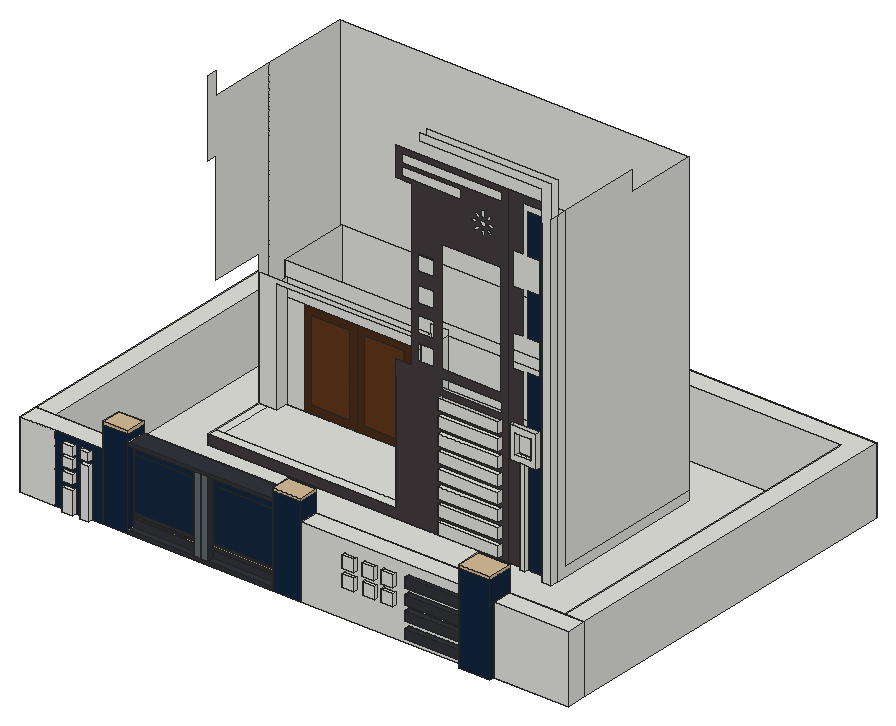
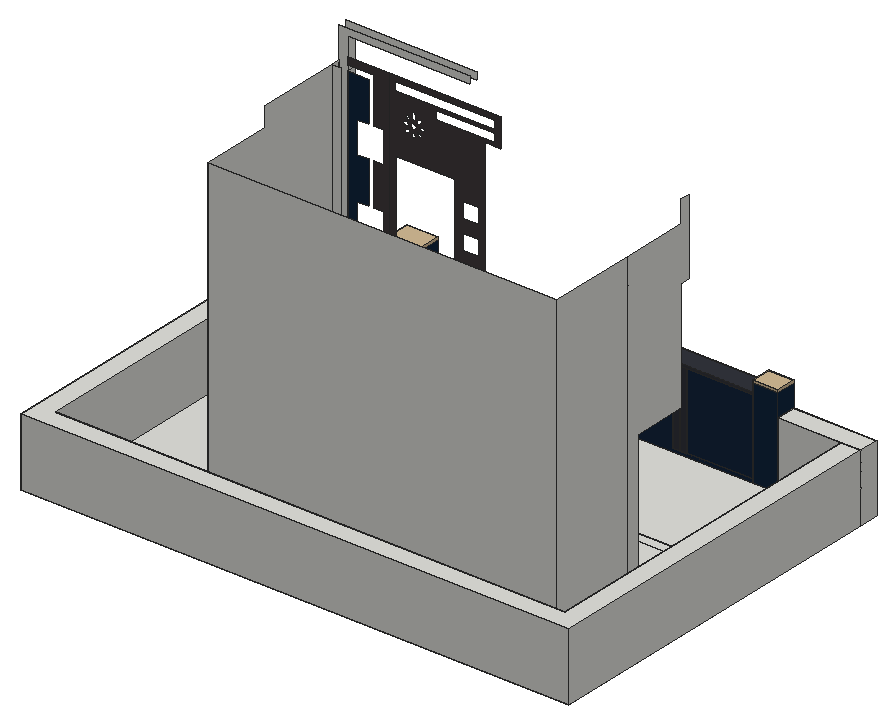
# SketchUp Ruby script. Lengths in inches.
U = 1.inch
M = Sketchup.active_model
def pt(a) = Geom::Point3d.new(a.map { |v| v * U })
def face(e, loops, mat)
  f = e.add_face(loops[0].map { |a| pt(a) })
  loops[1..].each { |l| e.add_face(l.map { |a| pt(a) }).erase! }
  f.material = f.back_material = mat if mat
  f
end
# faces: each face lists its corners as indices into pts; further lists are holes
def faces(e, pts, list, mat = nil) = list.each { |f| face(e, (f[0].is_a?(Array) ? f : [f]).map { |l| l.map { |i| pts[i] } }, mat) }
# xy, xz, yz: faces in a plane at the given z, y or x. An outline is a flat list of corners, or four numbers for a rectangle; further outlines are holes
def ring(l) = l.size == 4 ? [[l[0], l[1]], [l[2], l[1]], [l[2], l[3]], [l[0], l[3]]] : l.each_slice(2).to_a
def flat(e, list, mat, &to3) = list.each { |f| face(e, (f[0].is_a?(Array) ? f : [f]).map { |l| ring(l).map { |u, v| to3.(u, v) } }, mat) }
def xy(e, z, list, mat = nil) = flat(e, list, mat) { |x, y| [x, y, z] }
def xz(e, y, list, mat = nil) = flat(e, list, mat) { |x, z| [x, y, z] }
def yz(e, x, list, mat = nil) = flat(e, list, mat) { |y, z| [x, y, z] }
def lines(e, pts, list) = list.each { |a, b| e.add_line(pt(pts[a]), pt(pts[b])) }
# prism: a flat outline (further loops are holes) pulled along v
def prism(e, loops, v, mat = nil)
  f = face(e, loops, mat); d = Geom::Vector3d.new(v.map { |x| x * U })
  f.pushpull(f.normal.samedirection?(d) ? d.length : -d.length)
end
def box(e, o, s, mat = nil) = prism(e, [[o, [o[0] + s[0], o[1], o[2]], [o[0] + s[0], o[1] + s[1], o[2]], [o[0], o[1] + s[1], o[2]]]], [0, 0, s[2]], mat)
def at(x, y, z, deg = 0) = Geom::Transformation.translation(pt([x, y, z])) * Geom::Transformation.rotation(ORIGIN, Z_AXIS, deg.degrees)
def axes(o, x, y, z) = Geom::Transformation.new([*x, 0, *y, 0, *z, 0, *pt(o).to_a, 1])
def part(name) = M.definitions.add(name)
# library, detail: a bought-in or finely detailed component or shape, given as its bounding box
def library(name, o, s) = part(name).tap { |d| box(d.entities, o, s) }
def detail(e, o, s) = box(e.add_group.entities, o, s)
def put(e, d, t, mat = nil) = e.add_instance(d, t).tap { |i| i.material = mat if mat }
def group(e, t, mat = nil) = e.add_group.tap { |g| g.transformation = t; g.material = mat if mat }.entities
root = M.entities
M.materials.add("[Asphalt New]").color = [96, 86, 89]
M.materials.add("[Asphalt New]1").color = [67, 60, 62]
M.materials.add("[Carrera Marble]").color = [19, 39, 63]
M.materials.add("[Carrera Marble]1").color = [22, 39, 63]
M.materials.add("[Formica Beige]").color = [211, 187, 149]
M.materials.add("[Formica Laminate Dark]").color = [50, 53, 60]
M.materials.add("[Formica Speckled Grey]").color = [94, 105, 111]
M.materials.add("[Wood Cherry Original]").color = [96, 54, 26]
M.materials.add("[Wood Veneer 01]").color = [76, 44, 23]
xy(root,-39.0625,[[433.06,0,463.46,24.21],[44.56,0.625,54.43,5],[61.81,0.625,70.31,5],[0,5,81.17,24.21],[81.17,5,105.62,24.21],
  [105.62,5,247.01,24.21],[247.01,5,274.33,24.21],[274.33,5,433.06,24.21],[463.46,5,536.875,24.21],[0,24.21,0,381.625,536.875,381.625,536.875,24.21,517.66,24.21,517.66,362.41,19.21,362.41,19.21,24.21],
  [[19.21,24.21,517.66,362.41],[374.5,148.04,379.09,152.35]],[399.65,143.85,408.27,152.35],[374.5,148.04,379.09,152.35],[65.99,152.35,408.27,313.28]])
xy(root,-35.83,[[294.43,147.85,353.36,152.35]])
xy(root,-35.625,[[169.86,5,176.72,24.21],[176.72,5,183.58,24.21],[105.62,11.68,169.86,24.21]])
xy(root,-35.625,[[105.62,5,169.86,11.68],[183.58,5,247.01,11.68]],"[Formica Laminate Dark]")
xy(root,-32.16,[[380.62,0,433.06,5]],"[Formica Laminate Dark]")
xy(root,-30.0625,[[65.99,152.35,249.72,161.35],[399.27,161.35,399.27,304.28,74.99,304.28,74.99,226.93,65.99,226.93,65.99,313.28,408.27,313.28,408.27,161.35],[65.99,161.35,74.99,214.25],[74.99,161.35,399.27,161.35,399.27,226.93,241.35,226.93,241.35,214.25,224.39,214.25,224.39,226.93,83.43,226.93,83.43,214.25,74.99,214.25],[65.99,214.25,74.99,226.93],
  [74.99,214.25,83.43,226.93],[224.39,214.25,241.35,226.93],[74.99,226.93,399.27,234.75],[74.99,234.75,399.27,304.28]])
xy(root,-25.15,[[294.43,147.85,353.36,152.35]])
xy(root,-23.16,[[380.62,0,433.06,5]],"[Formica Laminate Dark]")
xy(root,-20.02,[[294.43,147.85,353.36,152.35]])
xy(root,-17.375,[[44.56,0.625,54.43,5]])
xy(root,-16.35,[[380.62,0,433.06,5]],"[Formica Laminate Dark]")
xy(root,-12.27,[[44.06,0.625,54.43,5]])
xy(root,-9.47,[[317.33,1.5625,329.02,5],[337.77,1.5625,349.45,5],[355.89,1.5625,367.58,5]])
xy(root,-9.33,[[294.43,147.85,353.36,152.35]])
xy(root,-7.35,[[380.62,0,433.06,5]],"[Formica Laminate Dark]")
xy(root,-4.33,[[294.43,147.85,353.36,152.35]])
xy(root,-3.45,[[44.06,0.625,54.43,5]])
xy(root,-2.54,[[380.62,0,433.06,5]],"[Formica Laminate Dark]")
xy(root,1.11,[[44.06,0.625,54.43,5]])
xy(root,2.22,[[317.33,1.5625,329.02,5],[337.77,1.5625,349.45,5],[355.89,1.5625,367.58,5]])
xy(root,6.35,[[294.43,147.85,353.36,152.35]])
xy(root,6.46,[[380.62,0,433.06,5]],"[Formica Laminate Dark]")
xy(root,7.16,[[317.33,1.5625,329.02,5],[337.45,1.5625,349.14,5],[355.95,1.5625,367.64,5]])
xy(root,9.75,[[61.81,0.625,70.31,5]])
xy(root,9.92,[[44.06,0.625,54.43,5]])
xy(root,11.17,[[294.43,147.85,353.36,152.35]])
xy(root,12.67,[[44.06,0.625,54.43,5]])
xy(root,12.9,[[380.62,0,433.06,5]],"[Formica Laminate Dark]")
xy(root,13.2,[[61.37,0.625,69.68,5]])
xy(root,18.84,[[317.33,1.5625,329.02,5],[337.45,1.5625,349.14,5],[355.95,1.5625,367.64,5]])
xy(root,21.48,[[44.06,0.625,54.43,5]])
xy(root,21.51,[[61.37,0.625,69.68,5]])
xy(root,21.85,[[294.43,147.85,353.36,152.35]])
xy(root,21.9,[[380.62,0,433.06,5]],"[Formica Laminate Dark]")
xy(root,26.67,[[294.43,147.85,353.36,152.35]])
xy(root,27,[[0,5,81.17,24.21],[463.46,5,536.875,24.21],[0,24.21,19.21,24.21,19.21,362.41,517.66,362.41,517.66,24.21,536.875,24.21,536.875,381.625,0,381.625]])
xy(root,30.5625,[[274.33,5,433.06,24.21]])
xy(root,37.35,[[294.43,147.85,353.36,152.35]])
xy(root,38.57,[[105.62,5,169.86,11.68],[176.72,5,183.58,24.21],[183.58,5,247.01,11.68]])
xy(root,41.45,[[105.62,5,247.01,24.21]],"[Formica Laminate Dark]")
xy(root,42.17,[[294.43,147.85,353.36,152.35]])
xy(root,48.5625,[[433.06,0,463.46,24.21],[81.17,5,105.62,24.21],[247.01,5,274.33,24.21]])
xy(root,51.5,[[433.06,0,463.46,24.21],[81.17,5,105.62,24.21],[247.01,5,274.33,24.21]],"[Formica Beige]")
xy(root,52.85,[[294.43,147.85,353.36,152.35]])
xy(root,54.85,[[364.57,148.04,374.5,152.35],[374.5,148.04,379.09,152.35],[379.09,148.04,390.63,152.35]])
xy(root,57.67,[[294.43,147.85,353.36,152.35]])
xy(root,60.36,[[370.09,148.04,374.5,152.35],[374.5,148.04,379.09,152.35],[379.09,148.04,385.11,152.35]])
xy(root,68.35,[[294.43,147.85,353.36,152.35]])
xy(root,73.17,[[294.43,147.85,353.36,152.35]])
xz(root,0,[[433.06,-39.0625,463.46,48.5625]],"[Carrera Marble]")
xz(root,0,[[433.06,48.5625,463.46,51.5]],"[Formica Beige]")
xz(root,0,[[380.62,-32.16,433.06,-23.16],[380.62,-16.35,433.06,-7.35],[380.62,-2.54,433.06,6.46],[380.62,12.9,433.06,21.9]],"[Formica Laminate Dark]")
xz(root,0.625,[[44.56,-39.0625,54.43,-17.375],[61.81,-39.0625,70.31,9.75],[44.06,-12.27,54.43,-3.45],[44.06,1.11,54.43,9.92],[44.06,12.67,54.43,21.48],
  [61.37,13.2,69.68,21.51]])
xz(root,1.5625,[[317.33,-9.47,329.02,2.22],[337.77,-9.47,349.45,2.22],[355.89,-9.47,367.58,2.22],[317.33,7.16,329.02,18.84],[337.45,7.16,349.14,18.84],
  [355.95,7.16,367.64,18.84]])
xz(root,5,[[0,-39.0625,33.95,27],[44.56,-39.0625,54.43,-17.375],[61.81,-39.0625,70.31,9.75],[[274.33,-39.0625,433.06,-39.0625,433.06,-32.16,380.62,-32.16,380.62,-23.16,433.06,-23.16,433.06,-16.35,380.62,-16.35,380.62,-7.35,433.06,-7.35,433.06,-2.54,380.62,-2.54,380.62,6.46,433.06,6.46,433.06,12.9,380.62,12.9,380.62,21.9,433.06,21.9,433.06,30.5625,274.33,30.5625],[317.33,7.16,329.02,18.84],[337.45,7.16,349.14,18.84],[355.95,7.16,367.64,18.84],[317.33,-9.47,329.02,2.22],[337.77,-9.47,349.45,2.22],[355.89,-9.47,367.58,2.22]],[463.46,-39.0625,536.875,27],
  [44.06,-12.27,54.43,-3.45],[317.33,-9.47,329.02,2.22],[337.77,-9.47,349.45,2.22],[355.89,-9.47,367.58,2.22],[44.06,1.11,54.43,9.92],
  [317.33,7.16,329.02,18.84],[337.45,7.16,349.14,18.84],[355.95,7.16,367.64,18.84],[44.06,12.67,54.43,21.48],[61.37,13.2,69.68,21.51]])
xz(root,5,[[[33.95,-39.0625,44.56,-39.0625,44.56,-17.375,54.43,-17.375,54.43,-39.0625,61.81,-39.0625,61.81,9.75,70.31,9.75,70.31,-39.0625,81.17,-39.0625,81.17,27,33.95,27],[44.06,-12.27,54.43,-3.45],[44.06,1.11,54.43,9.92],[44.06,12.67,54.43,21.48],[61.37,13.2,69.68,21.51]],[81.17,-39.0625,105.62,48.5625],[247.01,-39.0625,274.33,48.5625]],"[Carrera Marble]")
xz(root,5,[[81.17,48.5625,105.62,51.5],[247.01,48.5625,274.33,51.5]],"[Formica Beige]")
xz(root,5,[[105.62,-39.0625,247.01,-35.625],[380.62,-32.16,433.06,-23.16],[380.62,-16.35,433.06,-7.35],[380.62,-2.54,433.06,6.46],[380.62,12.9,433.06,21.9],
  [105.62,38.57,247.01,41.45]],"[Formica Laminate Dark]")
xz(root,5,[[169.86,-35.625,176.72,38.57],[176.72,-35.625,183.58,38.57]],"[Formica Speckled Grey]")
xz(root,11.68,[[105.62,-22.46,169.86,28.43],[183.58,-22.46,247.01,28.43],[105.62,28.43,169.86,38.57],[183.58,28.43,247.01,38.57]],"[Carrera Marble]1")
xz(root,11.68,[[183.58,-29.53,247.01,-28.67],[105.62,-28.67,169.86,-27.39],[183.58,-25.97,247.01,-24.3],[105.62,-25.93,169.86,-25.04]],"[Formica Beige]")
xz(root,11.68,[[105.62,-35.625,169.86,-28.67],[183.58,-35.625,247.01,-29.53],[183.58,-28.67,247.01,-25.97],[105.62,-27.39,169.86,-25.93],[105.62,-25.04,169.86,-22.46],
  [183.58,-24.3,247.01,-22.46]],"[Formica Laminate Dark]")
xz(root,24.21,[[0,-39.0625,19.21,27],[19.21,-39.0625,81.17,27],[274.33,-39.0625,433.06,30.5625],[463.46,-39.0625,517.66,27],[517.66,-39.0625,536.875,27]])
xz(root,24.21,[[81.17,-39.0625,105.62,48.5625],[247.01,-39.0625,274.33,48.5625],[433.06,-39.0625,463.46,48.5625]],"[Carrera Marble]")
xz(root,24.21,[[105.62,-39.0625,105.62,-35.625,183.58,-35.625,183.58,38.57,247.01,38.57,247.01,-39.0625],[105.62,-35.625,169.86,38.57]],"[Carrera Marble]1")
xz(root,24.21,[[81.17,48.5625,105.62,51.5],[247.01,48.5625,274.33,51.5],[433.06,48.5625,463.46,51.5]],"[Formica Beige]")
xz(root,24.21,[[169.86,-35.625,176.72,38.57],[176.72,-35.625,183.58,38.57],[105.62,38.57,247.01,41.45]],"[Formica Laminate Dark]")
xz(root,143.85,[[399.65,-39.0625,408.27,-39.0625,408.27,313.1875,280.02,313.1875,280.02,306.375,399.65,306.375]])
xz(root,147.85,[[294.43,-35.83,353.36,-25.15],[294.43,-20.02,353.36,-9.33],[294.43,-4.33,353.36,6.35],[294.43,11.17,353.36,21.85],[294.43,26.67,353.36,37.35],
  [294.43,42.17,353.36,52.85],[294.43,57.67,353.36,68.35],[294.43,73.17,353.36,83.85]])
xz(root,148.04,[[374.5,-39.0625,379.09,54.85],[[364.57,54.85,390.63,85.66],[370.09,60.36,385.11,80.14]]])
xz(root,152.35,[[399.65,-39.0625,399.65,306.375,280.02,306.375,280.02,313.1875,408.27,313.1875,408.27,-39.0625],[374.5,-39.0625,379.09,54.85],[294.43,-35.83,353.36,-25.15],[294.43,-20.02,353.36,-9.33],[294.43,-4.33,353.36,6.35],
  [294.43,11.17,353.36,21.85],[294.43,26.67,353.36,37.35],[294.43,42.17,353.36,52.85],[[364.57,54.85,390.63,85.66],[370.09,60.36,385.11,80.14]],[294.43,57.67,353.36,68.35],
  [370.09,60.36,385.11,80.14],[294.43,73.17,353.36,83.85]])
xz(root,152.35,[[[65.99,-39.0625,359.04,-39.0625,359.04,288.3125,249.72,288.3125,249.72,260.08,265.65,260.08,265.65,101,249.72,101,249.72,-30.0625,65.99,-30.0625],[295.03,107.34,352.78,217.65],[255.42,274.4,353.17,283.34],[294.43,57.67,353.36,68.35],[294.43,-20.02,353.36,-9.33],[294.43,26.67,353.36,37.35],[294.43,73.17,353.36,83.85],[294.43,88.67,353.36,99.35],[294.43,-35.83,353.36,-25.15],[294.43,42.17,353.36,52.85],[294.43,-4.33,353.36,6.35],[294.43,11.17,353.36,21.85],[255.42,262.6875,313.23,271.625],[271.51,157.4,287.33,173.21],[271.51,106.65,287.33,122.46],[271.51,185.28,287.33,201.09],[271.51,131.4,287.33,147.21],[334.77,253.73,334.15,254.28,333.625,254.91,333.2,255.62,332.89,256.39,332.7,257.1875,332.64,258.01,332.7,258.83,332.89,259.64,333.2,260.4,333.625,261.11,334.15,261.74,334.77,262.29,335.45,261.78,336.03,261.16,336.51,260.46,336.85,259.68,337.07,258.86,337.14,258.01,337.07,257.16,336.85,256.34,336.51,255.5625,336.03,254.86,335.45,254.24],[335.16,246.57,334.45,246.66,333.78,246.9375,333.21,247.375,332.78,247.95,332.5,248.61,332.41,249.32,332.5,250.03,332.78,250.7,333.21,251.26,333.78,251.7,334.45,251.98,335.16,252.07,335.87,251.98,336.53,251.7,337.1,251.26,337.54,250.7,337.8125,250.03,337.91,249.32,337.8125,248.61,337.54,247.95,337.1,247.375,336.53,246.9375,335.87,246.66],[342.77,247.64,342.04,247.7,341.33,247.88,340.68,248.18,340.1,248.58,339.62,249.07,339.25,249.63,339.62,250.2,340.1,250.6875,340.68,251.09,341.33,251.39,342.04,251.57,342.77,251.63,343.5,251.57,344.2,251.39,344.85,251.09,345.43,250.6875,345.91,250.2,346.28,249.63,345.91,249.07,345.43,248.58,344.85,248.18,344.2,247.88,343.5,247.7],[331.37,252.53,330.72,252.54,330.08,252.65,329.46,252.85,328.88,253.14,328.35,253.52,327.89,253.98,327.5,254.5,327.1875,255.07,326.97,255.68,326.85,256.32,326.83,256.97,327.5,257.27,328.21,257.42,328.94,257.43,329.66,257.29,330.33,257.01,330.9375,256.6,331.45,256.08,331.84,255.47,332.1,254.78,332.22,254.0625,332.1875,253.33,332.01,252.625],[326.94,247.92,326.07,247.99,325.22,248.18,324.43,248.49,323.7,248.91,323.08,249.43,323.52,249.97,324.07,250.4375,324.71,250.82,325.41,251.1,326.17,251.27,326.94,251.33,327.72,251.27,328.47,251.1,329.18,250.82,329.8125,250.4375,330.36,249.97,330.81,249.43,330.18,248.91,329.46,248.49,328.66,248.18,327.82,247.99],[342.9,240.98,342.24,241.01,341.6,241.15,340.99,241.375,340.41,241.7,339.9,242.1,339.45,242.58,339.08,243.125,338.8,243.72,338.61,244.35,338.52,245,338.53,245.65,339.2,245.81,339.89,245.84,340.57,245.75,341.23,245.55,341.84,245.23,342.38,244.8125,342.85,244.31,343.22,243.73,343.48,243.09,343.62,242.42,343.65,241.73,343.55,241.05],[326.99,241.29,326.25,241.35,326.4375,242.06,326.7,242.73,327.05,243.37,327.48,243.96,327.97,244.5,328.53,244.97,329.14,245.37,329.79,245.69,330.48,245.93,331.19,246.09,331.92,246.15,332.64,246.13,332.5,245.4,332.25,244.71,331.92,244.05,331.5,243.4375,331.01,242.89,330.45,242.4,329.83,242,329.16,241.68,328.46,241.46,327.73,241.32],[335.02,238.02,334.5625,238.48,334.17,239.01,333.86,239.57,333.63,240.18,333.5,240.81,333.45,241.45,333.5,242.09,333.63,242.72,333.86,243.33,334.17,243.9,334.5625,244.42,335.02,244.88,335.59,244.48,336.08,243.99,336.48,243.42,336.77,242.8,336.94,242.13,337,241.45,336.94,240.77,336.77,240.11,336.48,239.49,336.08,238.92,335.59,238.43],[338.82,252.65,338.71,253.3125,338.7,253.99,338.79,254.65,338.98,255.3,339.27,255.91,339.64,256.47,340.1,256.97,340.62,257.39,341.2,257.73,341.83,257.98,342.49,258.13,343.16,258.19,343.2,257.48,343.14,256.77,342.97,256.07,342.71,255.41,342.36,254.8,341.92,254.24,341.4,253.74,340.82,253.33,340.19,253.01,339.52,252.78]],[359.04,-39.0625,374.5,-39.0625,374.5,54.85,364.57,54.85,364.57,85.66,374.5,85.66,374.5,133.35,364.57,133.35,364.57,164.16,374.5,164.16,374.5,205.28,364.57,205.28,364.57,236.1,374.5,236.1,374.5,281.1,399.65,281.1,399.65,288.3125,359.04,288.3125]],"[Asphalt New]1")
xz(root,152.35,[[379.09,-39.0625,399.65,-39.0625,399.65,275.21,379.09,275.21,379.09,236.1,390.63,236.1,390.63,205.28,379.09,205.28,379.09,164.16,390.63,164.16,390.63,133.35,379.09,133.35,379.09,85.66,390.63,85.66,390.63,54.85,379.09,54.85]],"[Carrera Marble]")
xz(root,161.35,[[249.72,-30.0625,399.27,84.875],[399.27,-30.0625,408.27,281.9375]])
xz(root,214.25,[[65.99,-30.0625,83.43,-30.0625,83.43,81.17,224.39,81.17,224.39,-30.0625,241.35,-30.0625,241.35,84.875,65.99,84.875]])
xz(root,226.93,[[83.43,-30.0625,99.8125,63.53],[204.63,-30.0625,224.39,63.53],[224.39,-30.0625,241.35,89.9375],[241.35,-30.0625,399.27,84.875],[83.43,63.53,224.39,81.17]])
xz(root,226.93,[[106.9375,-22.9375,145.1,56.41],[159.35,-22.9375,197.5,56.41]],"[Wood Cherry Original]")
xz(root,226.93,[[[99.8125,-30.0625,152.22,63.53],[106.9375,-22.9375,145.1,56.41]],[[152.22,-30.0625,204.63,63.53],[159.35,-22.9375,197.5,56.41]]],"[Wood Veneer 01]")
xz(root,234.75,[[74.99,-30.0625,399.27,89.9375]])
xz(root,304.28,[[74.99,-30.0625,399.27,89.9375]])
xz(root,313.28,[[65.99,-39.0625,408.27,-30.0625],[65.99,-30.0625,408.27,262.6875]])
xz(root,362.41,[[19.21,-39.0625,517.66,27]])
xz(root,381.625,[[0,-39.0625,536.875,27]])
yz(root,0,[[5,-39.0625,24.21,27],[24.21,-39.0625,381.625,27]])
yz(root,19.21,[[24.21,-39.0625,362.41,27]])
yz(root,44.06,[[0.625,-12.27,5,-3.45],[0.625,1.11,5,9.92],[0.625,12.67,5,21.48]])
yz(root,44.56,[[0.625,-39.0625,5,-17.375]])
yz(root,54.43,[[0.625,-39.0625,5,-17.375],[0.625,-12.27,5,-3.45],[0.625,1.11,5,9.92],[0.625,12.67,5,21.48]])
yz(root,61.37,[[0.625,13.2,5,21.51]])
yz(root,61.81,[[0.625,-39.0625,5,9.75]])
yz(root,65.99,[[152.35,-39.0625,313.28,-30.0625],[214.25,-30.0625,214.25,101,161.35,101,161.35,209.9375,152.35,209.9375,152.35,284.4375,161.35,284.4375,161.35,262.6875,226.93,262.6875,226.93,-30.0625],[226.93,-30.0625,313.28,262.6875]])
yz(root,69.68,[[0.625,13.2,5,21.51]])
yz(root,70.31,[[0.625,-39.0625,5,9.75]])
yz(root,74.99,[[234.75,-30.0625,304.28,89.9375]])
yz(root,81.17,[[5,-39.0625,24.21,27]])
yz(root,81.17,[[5,27,24.21,48.5625]],"[Carrera Marble]")
yz(root,81.17,[[5,48.5625,24.21,51.5]],"[Formica Beige]")
yz(root,83.43,[[214.25,-30.0625,226.93,81.17]])
yz(root,105.62,[[5,-39.0625,24.21,-35.625],[11.68,-35.625,24.21,38.57],[5,38.57,24.21,41.45]])
yz(root,105.62,[[5,41.45,24.21,48.5625]],"[Carrera Marble]")
yz(root,105.62,[[5,-35.625,11.68,38.57]],"[Carrera Marble]1")
yz(root,105.62,[[5,48.5625,24.21,51.5]],"[Formica Beige]")
yz(root,169.86,[[11.68,-35.625,24.21,38.57]])
yz(root,169.86,[[5,-35.625,11.68,38.57]],"[Formica Laminate Dark]")
yz(root,176.72,[[5,-35.625,24.21,38.57]])
yz(root,183.58,[[11.68,-35.625,24.21,38.57]])
yz(root,183.58,[[5,-35.625,11.68,38.57]],"[Formica Laminate Dark]")
yz(root,224.39,[[214.25,-30.0625,226.93,81.17]])
yz(root,241.35,[[214.25,-30.0625,226.93,84.875]])
yz(root,247.01,[[5,-39.0625,5,-35.625,11.68,-35.625,11.68,38.57,24.21,38.57,24.21,-39.0625],[5,38.57,24.21,41.45]])
yz(root,247.01,[[5,41.45,24.21,48.5625]],"[Carrera Marble]")
yz(root,247.01,[[5,-35.625,11.68,38.57]],"[Carrera Marble]1")
yz(root,247.01,[[5,48.5625,24.21,51.5]],"[Formica Beige]")
yz(root,249.72,[[152.35,-30.0625,161.35,84.875]],"[Asphalt New]")
yz(root,274.33,[[5,-39.0625,24.21,30.5625]])
yz(root,274.33,[[5,30.5625,24.21,48.5625]],"[Carrera Marble]")
yz(root,274.33,[[5,48.5625,24.21,51.5]],"[Formica Beige]")
yz(root,294.43,[[147.85,-35.83,152.35,-25.15],[147.85,-20.02,152.35,-9.33],[147.85,-4.33,152.35,6.35],[147.85,11.17,152.35,21.85],[147.85,26.67,152.35,37.35],
  [147.85,42.17,152.35,52.85],[147.85,57.67,152.35,68.35],[147.85,73.17,152.35,83.85]])
yz(root,317.33,[[1.5625,-9.47,5,2.22],[1.5625,7.16,5,18.84]])
yz(root,329.02,[[1.5625,-9.47,5,2.22],[1.5625,7.16,5,18.84]])
yz(root,337.45,[[1.5625,7.16,5,18.84]])
yz(root,337.77,[[1.5625,-9.47,5,2.22]])
yz(root,349.14,[[1.5625,7.16,5,18.84]])
yz(root,349.45,[[1.5625,-9.47,5,2.22]])
yz(root,353.36,[[147.85,-35.83,152.35,-25.15],[147.85,-20.02,152.35,-9.33],[147.85,-4.33,152.35,6.35],[147.85,11.17,152.35,21.85],[147.85,26.67,152.35,37.35],
  [147.85,42.17,152.35,52.85],[147.85,57.67,152.35,68.35],[147.85,73.17,152.35,83.85]])
yz(root,355.89,[[1.5625,-9.47,5,2.22]])
yz(root,355.95,[[1.5625,7.16,5,18.84]])
yz(root,364.57,[[148.04,54.85,152.35,85.66]])
yz(root,367.58,[[1.5625,-9.47,5,2.22]])
yz(root,367.64,[[1.5625,7.16,5,18.84]])
yz(root,370.09,[[148.04,60.36,152.35,80.14]])
yz(root,374.5,[[148.04,-39.0625,152.35,54.85]])
yz(root,379.09,[[148.04,-39.0625,152.35,54.85]])
yz(root,380.62,[[0,-32.16,5,-23.16],[0,-16.35,5,-7.35],[0,-2.54,5,6.46],[0,12.9,5,21.9]],"[Formica Laminate Dark]")
yz(root,385.11,[[148.04,60.36,152.35,80.14]])
yz(root,390.63,[[148.04,54.85,152.35,85.66]])
yz(root,399.27,[[161.35,-30.0625,226.93,84.875],[226.93,-30.0625,234.75,89.9375],[234.75,-30.0625,304.28,89.9375]])
yz(root,399.65,[[143.85,-39.0625,152.35,275.21]])
yz(root,408.27,[[143.85,-39.0625,152.35,281.9375],[152.35,-39.0625,313.28,-39.0625,313.28,-30.0625,161.35,-30.0625,161.35,281.9375,152.35,281.9375],[161.35,-30.0625,313.28,-30.0625,313.28,262.6875,243.33,262.6875,243.33,281.9375,161.35,281.9375]])
yz(root,433.06,[[5,-39.0625,24.21,30.5625]])
yz(root,433.06,[[0,-39.0625,5,-32.16],[0,-32.16,5,-23.16],[0,-23.16,5,-16.35],[0,-16.35,5,-7.35],[0,-7.35,5,-2.54],
  [0,-2.54,5,6.46],[0,6.46,5,12.9],[0,12.9,5,21.9],[0,21.9,5,30.5625],[0,30.5625,24.21,48.5625]],"[Carrera Marble]")
yz(root,433.06,[[0,48.5625,24.21,51.5]],"[Formica Beige]")
yz(root,463.46,[[5,-39.0625,24.21,27]])
yz(root,463.46,[[0,-39.0625,5,27],[0,27,24.21,48.5625]],"[Carrera Marble]")
yz(root,463.46,[[0,48.5625,24.21,51.5]],"[Formica Beige]")
yz(root,517.66,[[24.21,-39.0625,362.41,27]])
yz(root,536.875,[[5,-39.0625,24.21,27],[24.21,-39.0625,381.625,27]])
